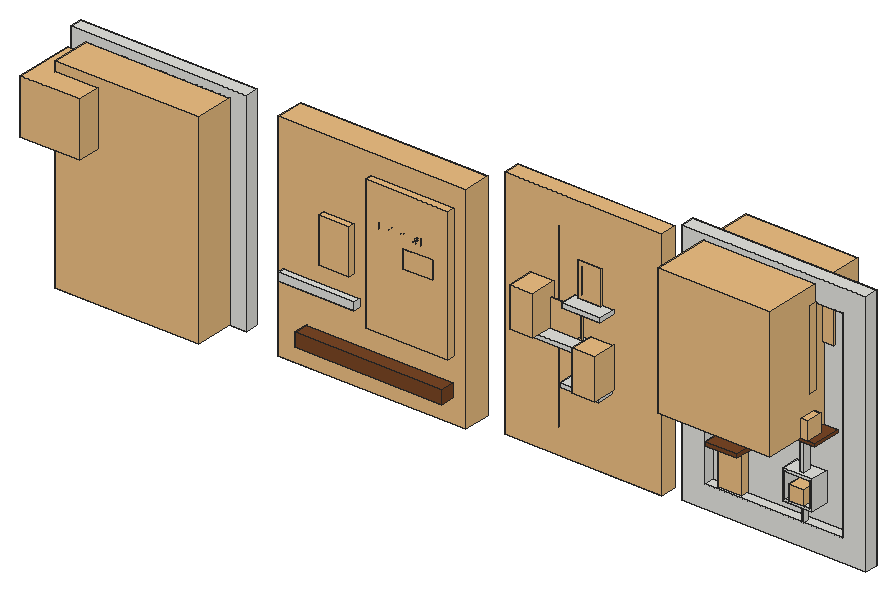
# SketchUp Ruby script. Lengths in inches.
U = 1.inch
M = Sketchup.active_model
def pt(a) = Geom::Point3d.new(a.map { |v| v * U })
def face(e, loops, mat)
  f = e.add_face(loops[0].map { |a| pt(a) })
  loops[1..].each { |l| e.add_face(l.map { |a| pt(a) }).erase! }
  f.material = f.back_material = mat if mat
  f
end
# faces: each face lists its corners as indices into pts; further lists are holes
def faces(e, pts, list, mat = nil) = list.each { |f| face(e, (f[0].is_a?(Array) ? f : [f]).map { |l| l.map { |i| pts[i] } }, mat) }
# xy, xz, yz: faces in a plane at the given z, y or x. An outline is a flat list of corners, or four numbers for a rectangle; further outlines are holes
def ring(l) = l.size == 4 ? [[l[0], l[1]], [l[2], l[1]], [l[2], l[3]], [l[0], l[3]]] : l.each_slice(2).to_a
def flat(e, list, mat, &to3) = list.each { |f| face(e, (f[0].is_a?(Array) ? f : [f]).map { |l| ring(l).map { |u, v| to3.(u, v) } }, mat) }
def xy(e, z, list, mat = nil) = flat(e, list, mat) { |x, y| [x, y, z] }
def xz(e, y, list, mat = nil) = flat(e, list, mat) { |x, z| [x, y, z] }
def yz(e, x, list, mat = nil) = flat(e, list, mat) { |y, z| [x, y, z] }
def lines(e, pts, list) = list.each { |a, b| e.add_line(pt(pts[a]), pt(pts[b])) }
# prism: a flat outline (further loops are holes) pulled along v
def prism(e, loops, v, mat = nil)
  f = face(e, loops, mat); d = Geom::Vector3d.new(v.map { |x| x * U })
  f.pushpull(f.normal.samedirection?(d) ? d.length : -d.length)
end
def box(e, o, s, mat = nil) = prism(e, [[o, [o[0] + s[0], o[1], o[2]], [o[0] + s[0], o[1] + s[1], o[2]], [o[0], o[1] + s[1], o[2]]]], [0, 0, s[2]], mat)
def at(x, y, z, deg = 0) = Geom::Transformation.translation(pt([x, y, z])) * Geom::Transformation.rotation(ORIGIN, Z_AXIS, deg.degrees)
def axes(o, x, y, z) = Geom::Transformation.new([*x, 0, *y, 0, *z, 0, *pt(o).to_a, 1])
def part(name) = M.definitions.add(name)
# library, detail: a bought-in or finely detailed component or shape, given as its bounding box
def library(name, o, s) = part(name).tap { |d| box(d.entities, o, s) }
def detail(e, o, s) = box(e.add_group.entities, o, s)
def put(e, d, t, mat = nil) = e.add_instance(d, t).tap { |i| i.material = mat if mat }
def group(e, t, mat = nil) = e.add_group.tap { |g| g.transformation = t; g.material = mat if mat }.entities
root = M.entities
M.materials.add("F5").color = [187, 207, 196]
M.materials.add("Material~12").color = [12, 12, 12]
M.materials.add("Material~27").color = [10, 10, 10]
M.materials.add("Material~28").color = [156, 145, 125]
M.materials.add("Material~29").color = [62, 62, 54]
M.materials.add("Material~42").color = [132, 97, 74]
M.materials.add("Material~43").color = [85, 62, 36]
M.materials.add("Querkus Oak Naturel Adagio _ Architonic1").color = [173, 130, 81]
M.materials.add("[Wood Veneer 01]").color = [120, 70, 37]
M.materials.add("mediterranean-hardwood-flooring").color = [114, 82, 60]
c1 = library("Potted foliage plant",[-34.87,-29.84,0],[109.95,108.62,128.4])
c2 = library("Potted succulent",[-1.34,0,0],[22.39,22.71,26.72])
c3 = library("Potted fan palm",[0,0,0],[52.56,47.17,54.17])
c4 = library("Group145\#1",[5.875,6.46,9.56],[20.8,10.13,11.36])
c5 = library("BOOJ",[0,0,0],[7.56,19.95,10.95])
c6 = library("Potted trailing philodendron",[-13.52,-13.75,-7.41],[40.56,40.5625,37.31])
c7 = library("PLANTS",[8.46,16.75,1.64],[23.16,16.42,22.13])
c8 = library("Buddha-Sitting[SKU_WDMG1527]\#1",[-16.46,-2.93,-0.22],[32.92,12.37,35.44])
c9 = library("Pot Nice",[-24.73,-24.73,-0.79],[49.46,49.46,53.07])
c10 = library("Desktop globe",[0,0,0],[12.93,11.94,21.27])
c11 = library("_CAPIM_DOS_PAMPAS_JULIAAIRES.3D",[-3.51,-2.78,-196.14],[35.86,35.18,43.25])
c12 = library("Potted croton",[2.12,-0.7,0],[25.93,26.45,60.75])
c13 = library("Group3\#1",[-226.43,63.68,0],[21.09,21.08,29.58])
c14 = library("Untitled (9)",[-9.61,-14.59,-0.92],[76.83,66.21,110.98])
c15 = library("Architecture and design books\#1",[9.67,-0.02,0],[20.02,11.1,12.25])
c16 = library("Potted Plant",[38.42,1.35,0],[44.68,49.99,41.74])
c17 = library("books",[6.19,-1.3125,-0.22],[15.35,11.9,12.07])
c18 = library("Livros",[0,0,0],[9.4375,8.82,3.7])
c19 = library("Ceiling Lamp 298 001",[-7.99,-7.99,-104.37],[15.97,15.98,104.68])
c20 = library("utensil 8",[0,0,0],[7.12,4.41,9.55])
c21 = library("Group\#2",[0,0,0],[128,19,146])
c22 = library("Group\#3",[-0.5,-0.5,0],[51.2,7,83.38])
c23 = library("Group\#6",[-0.5,-0.5,0],[1,1.55,124])
c24 = library("Group\#7",[0,0,0],[107,11,160])
c25 = library("Group\#9",[0,0,0],[16.02,5,137.29])
c26 = library("Group\#11",[0,0,0],[42.02,14,76])
c27 = part("3DGeom~6_Defintion")
xy(c27.entities,0,[[-470.59,-643.09,-470.4,291.53,529.41,291.53],[-470.59,-643.09,529.41,291.53,529.22,-643.09]])
xy(c27.entities,11.05,[[-470.59,-643.09,529.22,-643.09,529.41,291.53],[-470.59,-643.09,529.41,291.53,-470.4,291.53]])
xz(c27.entities,-643.09,[[-470.59,0,529.22,0,529.22,11.05],[-470.59,0,529.22,11.05,-470.59,11.05]])
xz(c27.entities,291.53,[[-470.4,0,-470.4,11.05,529.41,0],[529.41,0,-470.4,11.05,529.41,11.05]])
p = [[-470.4,291.53,0],[-470.59,-643.09,0],[-470.59,-643.09,11.05],[-470.4,291.53,11.05],[529.22,-643.09,0],[529.41,291.53,0],
  [529.41,291.53,11.05],[529.22,-643.09,11.05]]
faces(c27.entities,p,[[0,1,2],[2,3,0],[4,5,6],[6,7,4]])
c28 = part("Group72\#2")
put(c28.entities,c27,axes([-1.26,-0.65,45.42],[0.01717,0,0],[0,0,0.01717],[0,-0.01512,0]),"Material~12")
c29 = part("Group71\#2")
put(c29.entities,c28,at(0,0,0))
c30 = part("3DGeom~7_Defintion")
xy(c30.entities,14.63,[[-469.76,-662.07,-453.03,-645.34,-469.55,277.5],[-469.76,-662.07,513.32,-645.34,-453.03,-645.34],[-469.76,-662.07,530.04,-662.07,513.32,-645.34],[530.04,-662.07,513.52,260.77,513.32,-645.34],[530.04,-662.07,530.24,277.5,513.52,260.77],
  [-453.03,-645.34,-452.83,260.77,-469.55,277.5],[-452.83,260.77,530.24,277.5,-469.55,277.5],[-452.83,260.77,513.52,260.77,530.24,277.5]])
xz(c30.entities,-645.34,[[-453.03,2.4375,-453.03,14.63,513.32,2.4375],[513.32,2.4375,-453.03,14.63,513.32,14.63]])
xz(c30.entities,260.77,[[-452.83,2.4375,513.52,14.63,-452.83,14.63],[-452.83,2.4375,513.52,2.4375,513.52,14.63]])
p = [[-452.83,260.77,14.63],[-453.03,-645.34,14.63],[-453.03,-645.34,2.4375],[-452.83,260.77,2.4375],[513.32,-645.34,14.63],[513.52,260.77,14.63],
  [513.52,260.77,2.4375],[513.32,-645.34,2.4375]]
faces(c30.entities,p,[[0,1,2],[2,3,0],[4,5,6],[6,7,4]])
c31 = part("Group74\#2")
put(c31.entities,c30,axes([-1.26,-0.81,45.42],[0.01556,0,0],[0,0,0.01556],[0,-0.0137,0]),"Material~27")
c32 = part("Group73\#2")
put(c32.entities,c31,at(0,0,0))
c33 = part("3DGeom~8_Defintion")
xy(c33.entities,0,[[-469.76,-662.07,-469.55,277.5,530.04,-662.07],[530.04,-662.07,-469.55,277.5,530.24,277.5]],"Material~28")
xz(c33.entities,-662.07,[[-469.76,0,530.04,0,530.04,14.63],[-469.76,0,530.04,14.63,-469.76,14.63]],"Material~28")
xz(c33.entities,277.5,[[-469.55,0,-469.55,14.63,530.24,0],[530.24,0,-469.55,14.63,530.24,14.63]],"Material~28")
p = [[-469.55,277.5,0],[-469.76,-662.07,0],[-469.76,-662.07,14.63],[-469.55,277.5,14.63],[530.04,-662.07,0],[530.24,277.5,0],
  [530.24,277.5,14.63],[530.04,-662.07,14.63]]
faces(c33.entities,p,[[0,1,2],[2,3,0],[4,5,6],[6,7,4]],"Material~28")
c34 = part("Group76\#2")
put(c34.entities,c33,axes([-1.26,-0.81,45.42],[0.01556,0,0],[0,0,0.01556],[0,-0.0137,0]),"Material~28")
c35 = part("Group75\#2")
put(c35.entities,c34,at(0,0,0))
c36 = part("3DGeom~9_Defintion")
xy(c36.entities,58.03,[[373.52,427.46,360.6,440.375,-562.79,427.64],[-562.79,427.64,360.6,440.375,-549.87,440.56],[360.6,1414.36,-562.79,1427.46,-549.87,1414.54],[360.6,1414.36,373.52,1427.28,-562.79,1427.46]],"Material~28")
c37 = part("Group78\#2")
put(c37.entities,c36,axes([-17.1,-0.65,40.73],[0,0,-0.01762],[0.01762,0,0],[0,-0.01552,0]),"Material~28")
c38 = part("Group77\#2")
put(c38.entities,c37,at(0,0,0))
c39 = part("3DGeom~10_Defintion")
xy(c39.entities,58.03,[[-471.35,-6.46,515.55,6.46,-458.43,6.46],[-471.35,-6.46,528.47,-6.46,515.55,6.46],[-458.25,916.93,515.73,916.93,-471.17,929.85],[515.73,916.93,528.65,929.85,-471.17,929.85]],"Material~28")
c40 = part("Group80\#2")
put(c40.entities,c39,axes([-1.26,-0.65,34.26],[0.01762,0,0],[0,0,0.01762],[0,-0.01552,0]),"Material~28")
c41 = part("Group79\#2")
put(c41.entities,c40,at(0,0,0))
c42 = part("3DGeom~11_Defintion")
xy(c42.entities,0,[[-471.35,-6.46,-458.43,6.46,515.55,6.46],[-471.35,-6.46,515.55,6.46,528.47,-6.46],[-458.25,916.93,-471.17,929.85,515.73,916.93],[515.73,916.93,-471.17,929.85,528.65,929.85]])
xz(c42.entities,-6.46,[[-471.35,0,528.47,0,528.47,58.03],[-471.35,0,528.47,58.03,-471.35,58.03]])
xz(c42.entities,6.46,[[-458.43,0,-458.43,58.03,515.55,0],[515.55,0,-458.43,58.03,515.55,58.03]])
xz(c42.entities,916.93,[[-458.25,0,515.73,0,-458.25,58.03],[515.73,0,515.73,58.03,-458.25,58.03]])
xz(c42.entities,929.85,[[-471.17,0,-471.17,58.03,528.65,58.03],[-471.17,0,528.65,58.03,528.65,0]])
p = [[-458.43,6.46,0],[-471.35,-6.46,0],[-471.35,-6.46,58.03],[-458.43,6.46,58.03],[528.47,-6.46,0],[515.55,6.46,0],
  [515.55,6.46,58.03],[528.47,-6.46,58.03],[-458.25,916.93,0],[-458.25,916.93,58.03],[-471.17,929.85,58.03],[-471.17,929.85,0],
  [528.65,929.85,0],[528.65,929.85,58.03],[515.73,916.93,58.03],[515.73,916.93,0]]
faces(c42.entities,p,[[0,1,2],[2,3,0],[4,5,6],[6,7,4],[8,9,10],[10,11,8],[12,13,14],[14,15,12]])
c43 = part("Group82\#2")
put(c43.entities,c42,axes([-1.26,-0.65,34.26],[0.01762,0,0],[0,0,0.01762],[0,-0.01552,0]),"Material~27")
c44 = part("Group81\#2")
put(c44.entities,c43,at(0,0,0))
c45 = part("3DGeom~12_Defintion")
xy(c45.entities,0,[[373.52,427.46,-562.79,427.64,360.6,440.375],[-562.79,427.64,-549.87,440.56,360.6,440.375],[360.6,1414.36,-549.87,1414.54,-562.79,1427.46],[360.6,1414.36,-562.79,1427.46,373.52,1427.28]])
p = [[-562.79,427.64,0],[373.52,427.46,0],[373.52,427.46,58.03],[-562.79,427.64,58.03],[373.52,427.46,0],[360.6,440.375,0],
  [360.6,440.375,58.03],[373.52,427.46,58.03],[-549.87,440.56,0],[-562.79,427.64,0],[-562.79,427.64,58.03],[-549.87,440.56,58.03],
  [360.6,440.375,0],[-549.87,440.56,0],[-549.87,440.56,58.03],[360.6,440.375,58.03],[360.6,1414.36,0],[360.6,1414.36,58.03],
  [-549.87,1414.54,58.03],[-549.87,1414.54,0],[373.52,1427.28,0],[373.52,1427.28,58.03],[360.6,1414.36,58.03],[360.6,1414.36,0],
  [-549.87,1414.54,0],[-549.87,1414.54,58.03],[-562.79,1427.46,58.03],[-562.79,1427.46,0],[-562.79,1427.46,0],[-562.79,1427.46,58.03],
  [373.52,1427.28,58.03],[373.52,1427.28,0]]
faces(c45.entities,p,[[0,1,2],[2,3,0],[4,5,6],[6,7,4],[8,9,10],[10,11,8],[12,13,14],[14,15,12],
  [16,17,18],[18,19,16],[20,21,22],[22,23,20],[24,25,26],[26,27,24],[28,29,30],[30,31,28]])
c46 = part("Group84\#2")
put(c46.entities,c45,axes([-17.1,-0.65,40.73],[0,0,-0.01762],[0.01762,0,0],[0,-0.01552,0]),"Material~27")
c47 = part("Group83\#2")
put(c47.entities,c46,at(0,0,0))
c48 = part("3DGeom~13_Defintion")
xy(c48.entities,2.52,[[-468.71,-667.68,531.09,-667.68,-468.5,269.8],[531.09,-667.68,531.29,269.8,-468.5,269.8]],"Material~29")
c49 = part("Group86\#2")
put(c49.entities,c48,axes([-1.26,-0.81,45.42],[0.01504,0,0],[0,0,0.01504],[0,-0.01324,0]),"Material~29")
c50 = part("Group85\#2")
put(c50.entities,c49,at(0,0,0))
c51 = part("3DGeom~26_Defintion")
xy(c51.entities,0,[[-114.39,-1113.87,-114.39,-322.61,885.61,-322.61],[-114.39,-1113.87,885.61,-322.61,885.61,-1113.87]],"Material~43")
xy(c51.entities,1.46,[[-114.39,-1113.87,885.61,-1113.87,885.61,-322.61],[-114.39,-1113.87,885.61,-322.61,-114.39,-322.61]],"Material~43")
xz(c51.entities,-1113.87,[[-114.39,0,885.61,0,885.61,1.46],[-114.39,0,885.61,1.46,-114.39,1.46]])
xz(c51.entities,-322.61,[[-114.39,0,-114.39,1.46,885.61,0],[885.61,0,-114.39,1.46,885.61,1.46]])
yz(c51.entities,-114.39,[[-1113.87,0,-1113.87,1.46,-322.61,0],[-322.61,0,-1113.87,1.46,-322.61,1.46]])
yz(c51.entities,885.61,[[-1113.87,0,-322.61,0,-322.61,1.46],[-1113.87,0,-322.61,1.46,-1113.87,1.46]])
c52 = part("Group112\#2")
put(c52.entities,c51,axes([4.57,-0.8,76.9375],[-0.02129,0,0],[0,0,0.02129],[0,-0.02099,0]),"Material~43")
c53 = part("Group111\#2")
put(c53.entities,c52,at(0,0,0))
c54 = part("3DGeom~27_Defintion")
yz(c54.entities,-149.11,[[-1058.59,0,-1056.71,31.11,-250.79,31.11],[-1058.59,0,-1058.59,29.78,-1056.71,31.11],[-1058.59,0,-250.79,31.11,-248.91,0],[-248.91,0,-250.79,31.11,-248.91,29.78]])
yz(c54.entities,-108.07,[[-1017.55,7.8,-289.57,7.8,-291.45,19.93],[-1017.55,7.8,-291.45,19.93,-1017.55,18.6],[-289.57,7.8,-289.57,18.6,-291.45,19.93],[-1017.55,18.6,-291.45,19.93,-1015.67,19.93]])
yz(c54.entities,809.85,[[-1017.55,7.8,-1015.67,19.93,-289.57,7.8],[-1017.55,7.8,-1017.55,18.6,-1015.67,19.93],[-289.57,7.8,-1015.67,19.93,-289.57,18.6],[-289.57,18.6,-1015.67,19.93,-291.45,19.93]])
yz(c54.entities,850.89,[[-1058.59,0,-1056.71,31.11,-1058.59,29.78],[-1058.59,0,-248.91,0,-1056.71,31.11],[-248.91,0,-250.79,31.11,-1056.71,31.11],[-248.91,0,-248.91,29.78,-250.79,31.11]])
p = [[-108.07,-291.45,19.93],[-149.11,-250.79,31.11],[-149.11,-1056.71,31.11],[-108.07,-1015.67,19.93],[809.85,-1015.67,19.93],[850.89,-1056.71,31.11],
  [850.89,-250.79,31.11],[809.85,-291.45,19.93]]
faces(c54.entities,p,[[0,1,2],[2,3,0],[4,5,6],[6,7,4]])
c55 = part("Group114\#1")
put(c55.entities,c54,axes([4.57,-0.61,76.9375],[-0.0234,0,0],[0,0,0.0234],[0,-0.02306,0]),"Material~42")
c56 = part("Group113\#2")
put(c56.entities,c55,at(0,0,0))
c57 = library("Group115\#1",[-15.34,-1.33,52.16],[23.4,0.72,18.95])
c58 = library("Group117\#1",[-14.38,-1.1,53.125],[21.48,0.31,17.03])
c59 = library("Group131\#1",[9.73,-1.54,45.77],[27.4,0.89,13.28])
c60 = library("Group151\#2",[-15.34,-1.54,73.65],[10.68,0.89,11.15])
c61 = library("Group163\#1",[39.48,-0.86,42.54],[14.46,0.21,21.6])
c62 = library("Group165\#1",[41.15,-0.72,44.11],[11.23,0.03,18.43])
c63 = library("Group173\#1",[38.89,-1.29,42],[15.62,0.47,22.73])
c64 = library("Group\#408",[-8.45,0,0],[43.88,32.57,13.98])
c65 = library("Group\#388",[0,403.15,0],[76.9,397.92,354.24])
c66 = library("Group\#612",[-1.11,-0.87,0],[7.59,7.6,5.76])
box(root,[221.91,11.47,104.85],[29,15,4],"[Wood Veneer 01]")
box(root,[153.34,11.47,49.37],[52,15,5])
box(root,[343.26,13.97,49.81],[26.4,13,2.87])
box(root,[317.6,12.47,75.14],[37.4,13,2.87])
box(root,[344.46,13.97,98.94],[26.4,13,2.87])
xy(root,16.44,[[168.78,6.47,268.78,26.47]],"[Wood Veneer 01]")
xy(root,16.8125,[[497.84,26.47,499.84,29.73]])
xy(root,25.44,[[168.78,6.47,268.78,26.47]],"[Wood Veneer 01]")
xy(root,28.83,[[[489.27,21.47,509.27,33.47],[497.84,26.47,499.84,29.73]]])
xy(root,30.33,[[490.78,21.47,507.77,33.47]])
xy(root,47.32,[[490.78,21.47,507.77,33.47]])
xy(root,48.83,[[[489.27,21.47,509.27,33.47],[498.36,24.34,501.36,29.34]]])
xy(root,73.83,[[498.36,24.34,501.36,29.34]])
xy(root,74.65,[[468.11,13.47,517.11,33.47]],"[Wood Veneer 01]")
xy(root,76.65,[[468.11,13.47,517.11,33.47]],"[Wood Veneer 01]")
xz(root,6.47,[[168.78,16.44,268.78,25.44]],"[Wood Veneer 01]")
xz(root,13.47,[[468.11,74.65,517.11,76.65]],"[Wood Veneer 01]")
xz(root,21.47,[[[489.27,28.83,509.27,48.83],[490.78,30.33,507.77,47.32]]])
xz(root,24.34,[[498.36,48.83,501.36,73.83]])
xz(root,26.47,[[168.78,16.44,268.78,25.44],[497.84,16.8125,499.84,28.83]])
xz(root,29.34,[[498.36,48.83,501.36,73.83]])
xz(root,29.73,[[497.84,16.8125,499.84,28.83]])
xz(root,33.47,[[[489.27,28.83,509.27,48.83],[490.78,30.33,507.77,47.32]],[490.78,30.33,507.77,47.32],[468.11,74.65,517.11,76.65]])
yz(root,168.78,[[6.47,16.44,26.47,25.44]],"[Wood Veneer 01]")
yz(root,268.78,[[6.47,16.44,26.47,25.44]],"[Wood Veneer 01]")
yz(root,468.11,[[13.47,74.65,33.47,76.65]],"[Wood Veneer 01]")
yz(root,489.27,[[21.47,28.83,33.47,48.83]])
yz(root,490.78,[[21.47,30.33,33.47,47.32]])
yz(root,497.84,[[26.47,16.8125,29.73,28.83]])
yz(root,498.36,[[24.34,48.83,29.34,73.83]])
yz(root,499.84,[[26.47,16.8125,29.73,28.83]])
yz(root,501.36,[[24.34,48.83,29.34,73.83]])
yz(root,507.77,[[21.47,30.33,33.47,47.32]])
yz(root,509.27,[[21.47,28.83,33.47,48.83]])
yz(root,517.11,[[13.47,74.65,33.47,76.65]],"[Wood Veneer 01]")
detail(root,[10.79,0,0],[97.64,26.47,138.34])
detail(root,[212.91,11.47,41.58],[56.38,15,90.68])
detail(root,[493.19,32.47,127.48],[22,1,21.96])
put(root,c1,axes([455.5,8.08,76.65],[0.69,0,0],[0,0.69,0],[0,0,0.69]))
put(root,c2,axes([47.75,4.72,83.17],[0.76,0,0],[0,0.76,0],[0,0,0.76]))
put(root,c3,axes([494.05,20.72,30.85],[0.19673,0,0],[0,0.20632,0],[0,0,0.18864]))
put(root,c4,at(7.3,4.77,30.01))
put(root,c5,axes([38.64,4.77,117.82],[0,2,0],[2.03752,0,0],[0,0,1.41]))
put(root,c6,at(13.09,-1.82,102.29))
put(root,c7,axes([76.72,-14.28,77.74],[0.81,0,0],[0,1,0],[0,0,0.74]))
put(root,c8,axes([94.03,18.96,117.91],[0.5382,0,0],[0,0.58,0],[0,0,0.4425]))
put(root,c9,axes([45.07,10.57,39.82],[0.25357,0,0],[0,0.3276,0],[0,0,0.2964]))
put(root,c10,axes([68.01,14.47,48.82],[0.64,0,0],[0,0.74,0],[0,0,0.53]))
put(root,c11,axes([182.54,13.35,207.62],[0.57987,0,0],[0,0.47819,0],[0,0,0.71174]))
put(root,c12,axes([370.37,29.27,52.68],[0,-0.72,0],[-0.5874,0,0],[0,0,0.45]),"mediterranean-hardwood-flooring")
put(root,c12,axes([329.76,27.67,78.01],[0,-0.72,0],[-0.5874,0,0],[0,0,0.45]),"mediterranean-hardwood-flooring")
put(root,c13,axes([151.65,-29.88,78.95],[0.59809,0,0],[0,0.6048,0],[0,0,0.42]))
put(root,c14,axes([86.83,7.29,98.55],[0.21903,0,0],[0,0.33,0],[0,0,0.17508]))
put(root,c15,at(228.88,11.47,86.65))
put(root,c15,at(482.94,13.47,76.65))
put(root,c16,axes([10.89,8.53,59.52],[0.2097,0,0],[0,0.21818,0],[0,0,0.25242]))
put(root,c17,at(81.29,9.47,59.52))
put(root,c18,axes([14.71,12.38,98.39],[1.612,0,0],[0,1.34,0],[0,0,1]))
put(root,c19,axes([505.14,23.69,153.94],[0.336,0,0],[0,0.3481,0],[0,0,0.5117]))
put(root,c20,axes([247.79,18.05,25.44],[1.8318,0,0],[0,1.81,0],[0,0,1.29]))
g1 = group(root,at(0,26.47,0))
box(g1,[0,0,0],[120,9,144])
put(root,c21,at(149.45,16.47,0))
put(root,c22,at(215.36,20.47,45.24))
put(root,c23,at(333.68,26.43,16.88))
put(root,c24,at(296.93,25.47,0))
g2 = group(root,at(416.69,26.47,1.46))
xy(g2,0,[[0,0,125,9]])
xy(g2,15.36,[[15.36,0,109.64,7]])
xy(g2,152.64,[[15.36,0,109.64,7]])
xy(g2,168,[[0,0,125,9]])
xz(g2,0,[[[0,0,125,168],[15.36,15.36,109.64,152.64]]])
xz(g2,7,[[15.36,15.36,109.64,152.64]])
xz(g2,9,[[0,0,125,168]])
yz(g2,0,[[0,0,9,168]])
yz(g2,15.36,[[0,15.36,7,152.64]])
yz(g2,109.64,[[0,15.36,7,152.64]])
yz(g2,125,[[0,0,9,168]])
put(root,c25,at(439.53,28.47,16.8125),"[Wood Veneer 01]")
g3 = group(root,at(439.53,18.47,45.73),"[Wood Veneer 01]")
prism(g3,[[[-1,9,0],[16.02,9,0],[16.02,15,0],[21.02,15,0],[21.02,0,0],[-1,0,0]]],[0,0,2.42])
put(root,c26,at(439.53,19.47,62.07),"[Wood Veneer 01]")
g4 = group(root,at(153.34,22.87,54.37))
xy(g4,0.5,[[0.5,0.3,18.5,0.6]])
xy(g4,24,[[0.5,0.3,18.5,0.6]])
xz(g4,0.3,[[0.5,0.5,18.5,24]],"F5")
xz(g4,0.6,[[0.5,0.5,18.5,24]])
yz(g4,0.5,[[0.3,0.5,0.6,24]])
yz(g4,18.5,[[0.3,0.5,0.6,24]])
g5 = group(g4,at(0,0,0),"Querkus Oak Naturel Adagio _ Architonic1")
prism(g5,[[[0,0.6,0],[0,0.6,24.5],[19,0.6,24.5],[19,0.6,0]],[[0.5,0.6,0.5],[18.5,0.6,0.5],[18.5,0.6,24],[0.5,0.6,24]]],[0,-0.6,0])
put(root,c29,at(94.52,14.34,5.21))
put(root,c32,at(94.52,14.34,5.21))
put(root,c35,at(94.52,14.34,5.21))
put(root,c38,at(94.52,14.34,5.21))
put(root,c41,at(94.52,14.34,5.21))
put(root,c44,at(94.52,14.34,5.21))
put(root,c47,at(94.52,14.34,5.21))
put(root,c50,at(94.52,14.34,5.21))
put(root,c53,at(343.98,23.28,25.84))
put(root,c56,at(343.98,23.28,25.84))
put(root,c57,at(343.98,23.28,25.84))
put(root,c58,at(343.98,23.28,25.84))
put(root,c59,at(212.32,21.4,62.55))
put(root,c60,at(456.41,29.01,-25.49))
put(root,c61,at(308.93,25.26,59.82))
put(root,c62,at(308.93,25.26,59.82))
put(root,c63,at(308.93,25.26,59.82))
g6 = group(root,at(-274.75,49.47,15.21))
put(g6,c64,axes([718.3,-21.47,100.38],[0.4514,0.00006,0.00006],[-0.00006,0,0.4331],[0.00008,-0.61,0]))
put(g6,c65,axes([306.03,-44.43,47.61],[0,0.03672,0],[0.03672,0,0],[0,0,0.03672]))
put(g6,c66,axes([311.82,-45.82,47.61],[0,1.16847,0],[1.16847,0,0],[0,0,1.16847]))
